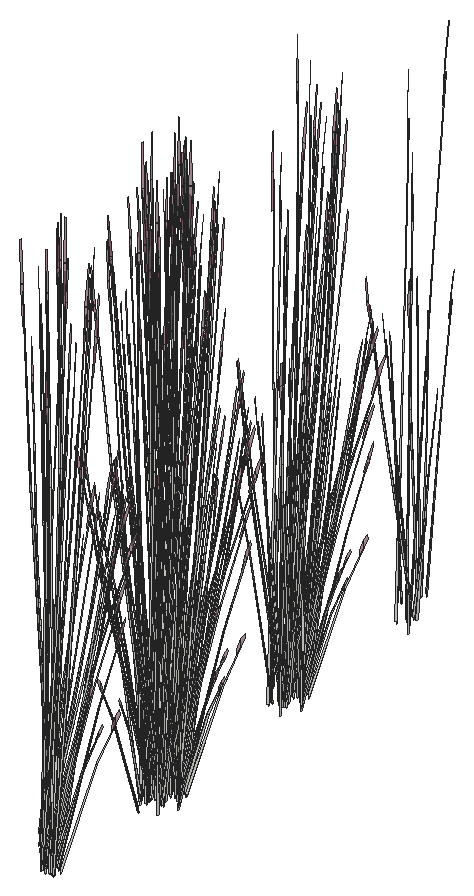
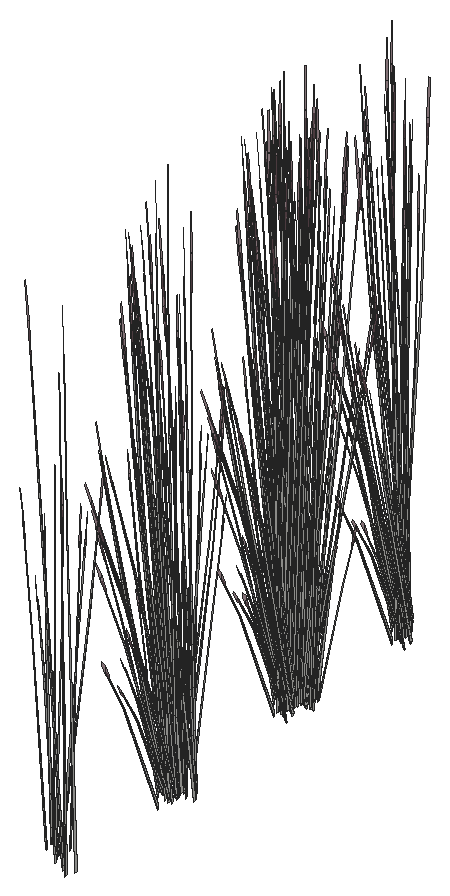
# SketchUp Ruby script. Lengths in inches.
U = 1.inch
M = Sketchup.active_model
def pt(a) = Geom::Point3d.new(a.map { |v| v * U })
def face(e, loops, mat)
  f = e.add_face(loops[0].map { |a| pt(a) })
  loops[1..].each { |l| e.add_face(l.map { |a| pt(a) }).erase! }
  f.material = f.back_material = mat if mat
  f
end
# faces: each face lists its corners as indices into pts; further lists are holes
def faces(e, pts, list, mat = nil) = list.each { |f| face(e, (f[0].is_a?(Array) ? f : [f]).map { |l| l.map { |i| pts[i] } }, mat) }
# xy, xz, yz: faces in a plane at the given z, y or x. An outline is a flat list of corners, or four numbers for a rectangle; further outlines are holes
def ring(l) = l.size == 4 ? [[l[0], l[1]], [l[2], l[1]], [l[2], l[3]], [l[0], l[3]]] : l.each_slice(2).to_a
def flat(e, list, mat, &to3) = list.each { |f| face(e, (f[0].is_a?(Array) ? f : [f]).map { |l| ring(l).map { |u, v| to3.(u, v) } }, mat) }
def xy(e, z, list, mat = nil) = flat(e, list, mat) { |x, y| [x, y, z] }
def xz(e, y, list, mat = nil) = flat(e, list, mat) { |x, z| [x, y, z] }
def yz(e, x, list, mat = nil) = flat(e, list, mat) { |y, z| [x, y, z] }
def lines(e, pts, list) = list.each { |a, b| e.add_line(pt(pts[a]), pt(pts[b])) }
# prism: a flat outline (further loops are holes) pulled along v
def prism(e, loops, v, mat = nil)
  f = face(e, loops, mat); d = Geom::Vector3d.new(v.map { |x| x * U })
  f.pushpull(f.normal.samedirection?(d) ? d.length : -d.length)
end
def box(e, o, s, mat = nil) = prism(e, [[o, [o[0] + s[0], o[1], o[2]], [o[0] + s[0], o[1] + s[1], o[2]], [o[0], o[1] + s[1], o[2]]]], [0, 0, s[2]], mat)
def at(x, y, z, deg = 0) = Geom::Transformation.translation(pt([x, y, z])) * Geom::Transformation.rotation(ORIGIN, Z_AXIS, deg.degrees)
def axes(o, x, y, z) = Geom::Transformation.new([*x, 0, *y, 0, *z, 0, *pt(o).to_a, 1])
def part(name) = M.definitions.add(name)
# library, detail: a bought-in or finely detailed component or shape, given as its bounding box
def library(name, o, s) = part(name).tap { |d| box(d.entities, o, s) }
def detail(e, o, s) = box(e.add_group.entities, o, s)
def put(e, d, t, mat = nil) = e.add_instance(d, t).tap { |i| i.material = mat if mat }
def group(e, t, mat = nil) = e.add_group.tap { |g| g.transformation = t; g.material = mat if mat }.entities
root = M.entities
M.materials.add("LightPink_Translucent").color = [144, 107, 117]
M.materials["LightPink_Translucent"].alpha = 0.75
c1 = part("blade")
p = [[2.15,0.21,22],[0,0.17,0],[0.09,0.45,0],[2.18,0.31,22],[2.29,0.31,22],[0.38,0.45,0],
  [2.48,0.24,33],[2.49,0.24,33],[2.48,0.22,33]]
faces(c1.entities,p,[[0,1,2,3],[4,5,2,3],[6,3,4,7],[8,0,3,6]])
c2 = part("seeds")
p = [[0.3,-0.1,1.38],[-0.01,-0.03,1.59],[-0.01,-0.03,0.03],[0.14,-0.07,-0.07],[0.29,-0.03,3],[0.15,0.01,3.11]]
faces(c2.entities,p,[[0,1,2,3],[1,0,4,5]],"LightPink_Translucent")
c3 = part("blade with seeds")
put(c3.entities,c1,at(0,0,0))
put(c3.entities,c2,axes([2.4,0.25,30.99],[1.5799,-0.05474,1.17369],[-0.12525,1.92788,0.29478],[-0.07173,-0.02425,1.56792]))
put(root,c3,axes([402.53,238.76,2.72],[0.38326,-0.02879,0.44739],[0.03466,0.47788,-0.21531],[-0.06861,0.04843,1.43643]))
put(root,c3,axes([402.77,238.28,2.62],[0.32884,-0.136,0.1448],[0.11516,0.38837,-0.41347],[0,0.08547,1.26744]))
put(root,c3,axes([403.99,239.22,2.59],[-0.085,-0.1147,1.43002],[0.1106,-0.37943,-0.30754],[0.17198,0.0514,0.61141]))
put(root,c3,axes([402.47,239.64,2.2],[0.35581,0.20937,0],[-0.17124,0.43505,0],[0,0,1.74954]))
put(root,c3,axes([402.61,240.1,2.19],[-0.21791,-0.46895,-0.05142],[0.36918,-0.26061,0.51607],[-0.09097,0.04465,1.6363]))
put(root,c3,axes([402.53,238.97,2.62],[0.26075,0.2802,0.1448],[-0.2175,0.31612,-0.41347],[-0.06054,0.04274,1.26744]))
put(root,c3,axes([403.21,239.45,4.98],[0.35281,0.01123,-0.71045],[-0.0237,0.47284,0.08574],[0.14947,0.0499,1.00501]))
put(root,c3,axes([402.8125,239.83,2.48],[0.33032,-0.23318,0.49651],[0.19744,0.41812,0],[-0.07523,0.05311,1.57504]))
put(root,c3,axes([402.34,239.46,2.29],[0.15345,0.53576,-0.06012],[-0.43845,0.18773,0],[0.00536,0.01871,1.72173]))
put(root,c3,axes([402.51,240.04,2.03],[-0.32928,-0.11539,-0.30978],[0.08291,-0.40636,0.30978],[-0.06638,0.04686,1.38974]))
put(root,c3,axes([403.78,238.49,2.375],[0.44133,0,0],[0,0.52122,-0.51607],[0,0.11871,1.63711]))
put(root,c3,axes([403.61,238.76,2.2],[-0.44111,-0.00373,-0.04976],[0,-0.52122,0.49943],[-0.01386,0.11865,1.58352]))
put(root,c3,axes([402.65,238.31,2.67],[0.39748,0.22252,-0.29095],[-0.19139,0.46966,-0.50002],[0.01249,0.11531,1.59708]))
put(root,c3,axes([403.42,239.65,4.53],[0.20082,0.29199,-0.35414],[-0.2293,0.2764,0.4572],[0.1165,0.04206,0.87481]))
put(root,c3,axes([403.52,238.84,2.03],[-0.24637,0.29097,-0.30978],[-0.24637,-0.29097,0.30978],[0,0.09372,1.38974]))
put(root,c3,axes([402.46,238.86,2.67],[0.04113,0.53214,-0.29095],[-0.42835,0.03218,-0.50002],[-0.07543,0.07088,1.59708]))
put(root,c3,axes([402.61,238.66,2.21],[-0.17124,0.42022,-0.44739],[-0.35581,-0.20224,0.21531],[0,0.09687,1.43643]))
put(root,c3,axes([402.62,239.86,2.33],[0.44186,0.15158,0.30756],[-0.11054,0.54181,-0.36492],[-0.07313,0.06781,1.64885]))
put(root,c3,axes([402.59,240.23,2.02],[-0.33032,0.23318,-0.49651],[-0.19744,-0.41812,0],[-0.07523,0.05311,1.57504]))
put(root,c3,axes([403.6875,238.85,2.02],[0,0.46636,-0.49651],[-0.39487,0,0],[0,0.10622,1.57504]))
put(root,c3,axes([402.7,238.9,3.875],[-0.1311,-0.08035,1.71376],[0.27131,-0.33708,0.13857],[0.16909,0.15206,0.73262]))
put(root,c3,axes([403.18,239.8125,2.77],[-0.19872,-0.13409,1.1486],[0.2566,-0.13625,0.84392],[0.06921,0.11541,0.25299]))
put(root,c3,axes([402.89,240.15,2.375],[0.22066,0.46731,0],[-0.36918,0.26061,-0.51607],[-0.08408,0.05936,1.63711]))
put(root,c3,axes([403.24,240.3125,1.49],[0.02571,-0.06733,1.76342],[0.32373,-0.19829,-0.26939],[0.09815,0.10263,0.30037]))
put(root,c3,axes([402.7,238.3,2.84],[-0.00964,-0.43909,1.41272],[0.43635,0.11382,0.59816],[-0.1032,0.24027,1.3335]))
put(root,c3,axes([402.8125,238.78,2.09],[0.12941,0.42699,-0.69212],[-0.37279,0.15378,-0.18165],[0.0143,0.14459,1.52773]))
put(root,c3,axes([402.74,240,4.68],[0.34827,-0.11086,-0.51099],[0.06092,0.41983,-0.3958],[0.09354,0.12031,0.97773]))
put(root,c3,axes([403.22,240.42,2.67],[-0.22633,-0.01463,1.0506],[0.14947,-0.31064,0.58006],[0.08941,0.11036,0.8241]))
put(root,c3,axes([402.48,239.67,2.59],[0.00623,-0.15459,1.43002],[0.29764,-0.17268,-0.30754],[0.09188,0.18503,0.61141]))
put(root,c3,axes([401.73,240.3,1.49],[0.05712,-0.02538,1.76342],[0.34359,0.13968,-0.26939],[0.01005,0.15742,0.30037]))
put(root,c3,axes([401.21,239.89,5],[0.25266,0.31335,-0.5672],[-0.2669,0.27442,-0.43934],[-0.03844,0.15921,1.08528]))
put(root,c3,axes([400.9375,240.36,2.82],[0.32063,-0.08258,0.06507],[0.07371,0.33271,-0.86304],[-0.02033,0.16842,0.7736]))
put(root,c3,axes([401.96,240.19,4.68],[0.34695,0.11691,-0.51099],[-0.11892,0.40083,-0.3958],[0.03181,0.16138,0.97773]))
put(root,c3,axes([402.16,239.37,3.875],[-0.08068,-0.14973,1.71376],[0.3728,-0.12606,0.13857],[0.08426,0.23506,0.73262]))
put(root,c3,axes([401.8,240.4375,4.53],[-0.1064,0.35863,-0.35414],[-0.31043,-0.1046,0.4572],[0.02846,0.14439,0.87481]))
put(root,c3,axes([401.5,239.44,3.875],[-0.00864,-0.17899,1.71376],[0.37441,0.11874,0.13857],[-0.02316,0.25508,0.73262]))
put(root,c3,axes([401.84,240.12,4.98],[0.16845,0.3792,-0.71045],[-0.34676,0.21133,0.08574],[0.03939,0.18322,1.00501]))
put(root,c3,axes([402.72,253.1,2.59],[-0.10032,0.0944,1.43002],[-0.30046,-0.16522,-0.30754],[0.05569,-0.20547,0.61141]))
put(root,c3,axes([402.27,253.42,4.98],[-0.16845,-0.3792,-0.71045],[0.34676,-0.21133,0.08574],[-0.03939,-0.18322,1.00501]))
put(root,c3,axes([401.98,252.58,1.49],[-0.0592,0.0168,1.76342],[-0.32738,-0.18913,-0.26939],[0.00549,-0.15776,0.30037]))
put(root,c3,axes([402.97,253.8,4.98],[0.00918,-0.43138,-0.71045],[0.38672,0.02897,0.08574],[0.04081,-0.18275,1.00501]))
put(root,c3,axes([402.3,253.1,4.53],[0.1064,-0.35863,-0.35414],[0.31043,0.1046,0.4572],[-0.02846,-0.14439,0.87481]))
put(root,c3,axes([402.53,253.58,3.875],[-0.06572,0.16029,1.71376],[-0.27569,-0.33172,0.13857],[0.12437,-0.20675,0.73262]))
put(root,c3,axes([402.14,253.35,4.68],[-0.34695,-0.11691,-0.51099],[0.11892,-0.40083,-0.3958],[-0.03181,-0.16138,0.97773]))
put(root,c3,axes([402.35,252.34,2.77],[0.04528,0.27194,1.1486],[-0.25117,-0.15062,0.84392],[0.02703,-0.13924,0.25299]))
put(root,c3,axes([402.89,253.65,4.68],[-0.25266,-0.31335,-0.51099],[0.2669,-0.27442,-0.3958],[0.03844,-0.15921,0.97773]))
put(root,c3,axes([403.13,253.54,4.53],[0.23881,-0.24554,-0.35414],[0.22606,0.28036,0.4572],[0.0344,-0.14245,0.87481]))
put(root,c3,axes([401.49,254.85,2.1],[-0.14494,-0.47823,-0.69835],[0.41752,-0.17223,-0.18329],[-0.01602,-0.16194,1.54149]))
put(root,c3,axes([403.43,253.39,1.49],[-0.05283,-0.03674,1.76342],[-0.13569,-0.41045,-0.26939],[0.09154,-0.11138,0.30037]))
put(root,c3,axes([403.42,254.55,4.98],[0.18436,-0.36797,-0.71045],[0.32306,0.26151,0.08574],[0.11008,-0.13332,1.00501]))
put(root,c3,axes([401.43,253.47,2.375],[-0.22066,-0.46731,0],[0.36918,-0.26061,-0.51607],[0.08408,-0.05936,1.63711]))
put(root,c3,axes([403.41,254.375,4.68],[-0.09067,-0.42583,-0.51099],[0.34336,-0.07449,-0.3958],[0.0984,-0.11438,0.97773]))
put(root,c3,axes([401.92,252.91,2.13],[-0.2439,0.26754,-0.03893],[-0.22348,-0.29302,-0.17649],[-0.01573,-0.08303,0.58215]))
put(root,c3,axes([400.63,254.78,2.02],[0,-0.46636,-0.49651],[0.39487,0,0],[0,-0.10622,1.57504]))
put(root,c3,axes([401.73,253.4,2.02],[0.33032,-0.23318,-0.49651],[0.19744,0.41812,0],[0.07523,-0.05311,1.57504]))
put(root,c3,axes([403.69,254.21,2.59],[-0.12609,-0.01381,1.43002],[-0.12917,-0.37055,-0.30754],[0.1549,-0.10482,0.61141]))
put(root,c3,axes([402.12,254.36,2.06],[0.23773,-0.35053,-0.62353],[0.29532,0.31785,-0.16365],[0.09526,-0.08744,1.37633]))
put(root,c3,axes([403.84,253.53,2.77],[-0.11756,0.2374,1.1486],[-0.10105,-0.31895,0.84392],[0.09709,-0.07992,0.25299]))
put(root,c3,axes([403.67,254.42,4.53],[0.30722,-0.06665,-0.35414],[0.08112,0.381,0.4572],[0.08804,-0.10234,0.87481]))
put(root,c3,axes([401.71,254.97,2.21],[0.17124,-0.42022,-0.44739],[0.35581,0.20224,0.21531],[0,-0.09687,1.43643]))
put(root,c3,axes([401.86,254.76,2.67],[-0.04113,-0.53214,-0.29095],[0.42835,-0.03218,-0.50002],[0.07543,-0.07088,1.59708]))
put(root,c3,axes([400.8,254.79,2.03],[0.24637,-0.29097,-0.30978],[0.24637,0.29097,0.30978],[0,-0.09372,1.38974]))
put(root,c3,axes([401.67,255.32,2.67],[-0.39748,-0.22252,-0.29095],[0.19139,-0.46966,-0.50002],[-0.01249,-0.11531,1.59708]))
put(root,c3,axes([401.81,253.59,2.03],[0.32928,0.11539,-0.30978],[-0.08291,0.40636,0.30978],[0.06638,-0.04686,1.38974]))
put(root,c3,axes([401.92,255.18,2.43],[0.39767,0.22603,0.24065],[-0.19139,0.46966,0.50002],[0,-0.10827,1.60543]))
put(root,c3,axes([401.77,255.82,2.4375],[0.09355,-0.55261,-0.23429],[0.44354,0.09633,0.51271],[-0.0775,-0.07631,1.5644]))
put(root,c3,axes([401.79,254.87,2.72],[-0.38326,0.02879,0.44739],[-0.03466,-0.47788,-0.21531],[0.06861,-0.04843,1.43643]))
put(root,c3,axes([400.8,255.22,2.48],[0,0.46636,0.49651],[-0.39487,0,0],[0,-0.10622,1.57504]))
put(root,c3,axes([403.57,255.32,4.68],[0.09562,-0.42421,-0.51099],[0.32782,0.1454,-0.3958],[0.13199,-0.0389,0.97773]))
put(root,c3,axes([403.06,253.59,2.375],[0.22066,-0.46731,0],[0.36918,0.26061,-0.51607],[0.08408,0.05936,1.63711]))
put(root,c3,axes([401.78,255.04,2.36],[0.15345,0.52148,0.45755],[-0.43845,0.18134,0.17955],[0.00536,-0.09582,1.58856]))
put(root,c3,axes([403.92,255.4375,1.98],[-0.22732,0.05597,1.41583],[-0.03618,-0.44548,0.08104],[0.15921,-0.06743,0.80566]))
put(root,c3,axes([404.34,255.04,2.26],[-0.21881,-0.29821,-0.06488],[0.23965,-0.27324,-0.29416],[0.0679,-0.01924,0.97024]))
put(root,c3,axes([401.7,255.45,2.72],[-0.17124,0.42022,0.44739],[-0.35581,-0.20224,-0.21531],[0,-0.09687,1.43643]))
put(root,c3,axes([402.33,255.08,2.21],[0,-0.53961,0],[0.44133,0,0],[0,0,1.79456]))
put(root,c3,axes([402.87,253.84,2.48],[-0.33032,-0.23318,0.49651],[0.19744,-0.41812,0],[0.07523,0.05311,1.57504]))
put(root,c3,axes([403.51,255.47,4.98],[0.31014,-0.20596,-0.71045],[0.17284,0.42397,0.08574],[0.14985,-0.04816,1.00501]))
put(root,c3,axes([402.12,254.74,2.36],[-0.29264,0.42323,0.45755],[-0.34767,-0.3736,0.17955],[0.07055,-0.04224,1.58856]))
put(root,c3,axes([402.44,255.5,2.3],[-0.32829,-0.4014,-0.06131],[0.32849,-0.40164,0],[-0.01146,-0.01402,1.75571]))
put(root,c3,axes([401.61,254.05,2.47],[-0.10196,0.46348,0.17642],[-0.3731,-0.13116,0.35086],[0.06445,-0.00226,1.60407]))
put(root,c3,axes([401.46,254.42,1.59],[-0.3474,0.18671,1.28929],[-0.11057,-0.53572,0.50096],[0.21332,0.00891,1.46642]))
put(root,c3,axes([402.39,254.5625,2.62],[0.06809,-0.4162,0.1448],[0.33266,0.07225,-0.41347],[0.06054,0.04274,1.26744]))
put(root,c3,axes([401.82,255.55,2.36],[0.44609,0.09826,0.45755],[-0.09078,0.55493,0.17955],[-0.06519,-0.05359,1.58856]))
put(root,c3,axes([404.17,255.15,1.49],[-0.01845,-0.0708,1.76342],[0.12793,-0.41416,-0.26939],[0.12905,-0.00596,0.30037]))
put(root,c3,axes([402.25,254.67,2.72],[-0.21202,-0.39143,0.44739],[0.32115,-0.27564,-0.21531],[0.06861,0.04843,1.43643]))
put(root,c3,axes([401.58,256.4375,2.47],[0.37926,-0.12378,0.17642],[0.09365,0.46065,0.35086],[-0.03382,-0.06712,1.60407]))
put(root,c3,axes([402.36,254.7,2.67],[0.35635,-0.30962,-0.29095],[0.23697,0.43749,-0.50002],[0.08792,0.04443,1.59708]))
put(root,c3,axes([403.78,255.51,4.53],[0.29332,0.1301,-0.35414],[-0.08555,0.37955,0.4572],[0.11809,-0.0348,0.87481]))
put(root,c3,axes([403.26,253.875,2.02],[0.33032,0.23318,-0.49651],[-0.19744,0.41812,0],[0.07523,0.05311,1.57504]))
put(root,c3,axes([402.63,255.2,2.21],[0.39487,0,0],[0,0.48281,0],[0,0,1.78407]))
put(root,c3,axes([402.74,254.07,2.47],[-0.37926,0.12378,0.17642],[-0.09365,-0.46065,0.35086],[0.03382,0.06712,1.60407]))
put(root,c3,axes([402.98,255.04,3.875],[-0.14639,0.01056,1.71376],[0.09712,-0.45778,0.13857],[0.20862,0.02831,0.73262]))
put(root,c3,axes([403.17,254.05,2.03],[0.08291,0.40636,-0.30978],[-0.32928,0.11539,0.30978],[0.06638,0.04686,1.38974]))
put(root,c3,axes([402.5,254.96,2.38],[-0.44609,-0.09826,0.49198],[0.09078,-0.55493,0.19306],[0.06519,0.05359,1.70813]))
put(root,c3,axes([402.15,256.33,2.2],[-0.11516,-0.40207,0],[0.32884,-0.1408,0],[0,0,1.54371]))
put(root,c3,axes([401.93,255.95,2.62],[-0.06809,0.4162,0.1448],[-0.33266,-0.07225,-0.41347],[-0.06054,-0.04274,1.26744]))
put(root,c3,axes([402.58,256.27,2.18],[0.37054,-0.15823,-0.19198],[0.1302,0.45581,0.00008],[0.0409,-0.01749,1.73897]))
put(root,c3,axes([402.71,256.46,2.47],[0.10196,-0.46348,0.17642],[0.3731,0.13116,0.35086],[-0.06445,0.00226,1.60407]))
put(root,c3,axes([402.62,255.41,2.21],[0.24637,0.30123,0],[-0.24637,0.30123,0],[0,0,1.69266]))
put(root,c3,axes([403.29,255.28,2.47],[-0.2773,-0.3397,0.17642],[0.27945,-0.32949,0.35086],[-0.03063,0.06937,1.60407]))
put(root,c3,axes([402.78,254.77,2.06],[0.36714,0.07646,-0.62353],[-0.07747,0.47163,-0.16365],[0.10956,0.05715,1.37633]))
put(root,c3,axes([404.4,255.59,2.77],[-0.21807,0.07699,1.1486],[0.10265,-0.31819,0.84392],[0.11568,0.02177,0.25299]))
put(root,c3,axes([402.07,256.51,2.2],[-0.35581,-0.20937,0],[0.17124,-0.43505,0],[0,0,1.62707]))
put(root,c3,axes([402.62,255.06,2.72],[0.17124,-0.42022,0.44739],[0.35581,0.20224,-0.21531],[0,0.09687,1.43643]))
put(root,c3,axes([402.55,255.3,2.29],[0,0.53934,-0.05637],[-0.44133,0,0],[0,0.01695,1.79368]))
put(root,c3,axes([402.58,254.92,2.21],[0.21202,0.39143,-0.44739],[-0.32115,0.27564,0.21531],[0.06861,0.04843,1.43643]))
put(root,c3,axes([404.02,256.57,3.93],[-0.06755,-0.39203,-0.03492],[0.31928,-0.09013,-0.15832],[0.06667,0.02485,0.52218]))
put(root,c3,axes([403.52,255.29,2.48],[0,-0.46636,0.49651],[0.39487,0,0],[0,0.10622,1.57504]))
put(root,c3,axes([402.53,255.64,2.72],[0.38326,-0.02879,0.44739],[0.03466,0.47788,-0.21531],[-0.06861,0.04843,1.43643]))
put(root,c3,axes([402.77,255.15,2.62],[0.32884,-0.136,0.1448],[0.11516,0.38837,-0.41347],[0,0.08547,1.26744]))
put(root,c3,axes([403.99,256.1,2.59],[-0.085,-0.1147,1.43002],[0.1106,-0.37943,-0.30754],[0.17198,0.0514,0.61141]))
put(root,c3,axes([402.47,256.52,2.2],[0.35581,0.20937,0],[-0.17124,0.43505,0],[0,0,1.74954]))
put(root,c3,axes([402.61,256.98,2.19],[-0.21791,-0.46895,-0.05142],[0.36918,-0.26061,0.51607],[-0.09097,0.04465,1.6363]))
put(root,c3,axes([402.53,255.85,2.62],[0.26075,0.2802,0.1448],[-0.2175,0.31612,-0.41347],[-0.06054,0.04274,1.26744]))
put(root,c3,axes([403.21,256.33,4.98],[0.35281,0.01123,-0.71045],[-0.0237,0.47284,0.08574],[0.14947,0.0499,1.00501]))
put(root,c3,axes([402.8125,256.71,2.48],[0.33032,-0.23318,0.49651],[0.19744,0.41812,0],[-0.07523,0.05311,1.57504]))
put(root,c3,axes([402.34,256.34,2.29],[0.15345,0.53576,-0.06012],[-0.43845,0.18773,0],[0.00536,0.01871,1.72173]))
put(root,c3,axes([402.51,256.92,2.03],[-0.32928,-0.11539,-0.30978],[0.08291,-0.40636,0.30978],[-0.06638,0.04686,1.38974]))
put(root,c3,axes([403.78,255.37,2.375],[0.44133,0,0],[0,0.52122,-0.51607],[0,0.11871,1.63711]))
put(root,c3,axes([403.61,255.64,2.2],[-0.44111,-0.00373,-0.04976],[0,-0.52122,0.49943],[-0.01386,0.11865,1.58352]))
put(root,c3,axes([402.65,255.19,2.67],[0.39748,0.22252,-0.29095],[-0.19139,0.46966,-0.50002],[0.01249,0.11531,1.59708]))
put(root,c3,axes([403.42,256.53,4.53],[0.20082,0.29199,-0.35414],[-0.2293,0.2764,0.4572],[0.1165,0.04206,0.87481]))
put(root,c3,axes([403.52,255.71,2.03],[-0.24637,0.29097,-0.30978],[-0.24637,-0.29097,0.30978],[0,0.09372,1.38974]))
put(root,c3,axes([402.46,255.74,2.67],[0.04113,0.53214,-0.29095],[-0.42835,0.03218,-0.50002],[-0.07543,0.07088,1.59708]))
put(root,c3,axes([402.61,255.53,2.21],[-0.17124,0.42022,-0.44739],[-0.35581,-0.20224,0.21531],[0,0.09687,1.43643]))
put(root,c3,axes([402.62,256.74,2.33],[0.44186,0.15158,0.30756],[-0.11054,0.54181,-0.36492],[-0.07313,0.06781,1.64885]))
put(root,c3,axes([402.59,257.11,2.02],[-0.33032,0.23318,-0.49651],[-0.19744,-0.41812,0],[-0.07523,0.05311,1.57504]))
put(root,c3,axes([403.6875,255.73,2.02],[0,0.46636,-0.49651],[-0.39487,0,0],[0,0.10622,1.57504]))
put(root,c3,axes([402.7,255.78,3.875],[-0.1311,-0.08035,1.71376],[0.27131,-0.33708,0.13857],[0.16909,0.15206,0.73262]))
put(root,c3,axes([403.18,256.69,2.77],[-0.19872,-0.13409,1.1486],[0.2566,-0.13625,0.84392],[0.06921,0.11541,0.25299]))
put(root,c3,axes([402.89,257.03,2.375],[0.22066,0.46731,0],[-0.36918,0.26061,-0.51607],[-0.08408,0.05936,1.63711]))
put(root,c3,axes([403.24,257.19,1.49],[0.02571,-0.06733,1.76342],[0.32373,-0.19829,-0.26939],[0.09815,0.10263,0.30037]))
put(root,c3,axes([402.7,255.18,2.84],[-0.00964,-0.43909,1.41272],[0.43635,0.11382,0.59816],[-0.1032,0.24027,1.3335]))
put(root,c3,axes([402.8125,255.66,2.09],[0.12941,0.42699,-0.69212],[-0.37279,0.15378,-0.18165],[0.0143,0.14459,1.52773]))
put(root,c3,axes([402.74,256.875,4.68],[0.34827,-0.11086,-0.51099],[0.06092,0.41983,-0.3958],[0.09354,0.12031,0.97773]))
put(root,c3,axes([403.22,257.3,2.67],[-0.22633,-0.01463,1.0506],[0.14947,-0.31064,0.58006],[0.08941,0.11036,0.8241]))
put(root,c3,axes([402.48,256.55,2.59],[0.00623,-0.15459,1.43002],[0.29764,-0.17268,-0.30754],[0.09188,0.18503,0.61141]))
put(root,c3,axes([401.73,257.18,1.49],[0.05712,-0.02538,1.76342],[0.34359,0.13968,-0.26939],[0.01005,0.15742,0.30037]))
put(root,c3,axes([401.21,256.77,5],[0.25266,0.31335,-0.5672],[-0.2669,0.27442,-0.43934],[-0.03844,0.15921,1.08528]))
put(root,c3,axes([400.9375,257.24,2.82],[0.32063,-0.08258,0.06507],[0.07371,0.33271,-0.86304],[-0.02033,0.16842,0.7736]))
put(root,c3,axes([401.96,257.07,4.68],[0.34695,0.11691,-0.51099],[-0.11892,0.40083,-0.3958],[0.03181,0.16138,0.97773]))
put(root,c3,axes([402.16,256.24,3.875],[-0.08068,-0.14973,1.71376],[0.3728,-0.12606,0.13857],[0.08426,0.23506,0.73262]))
put(root,c3,axes([401.8,257.32,4.53],[-0.1064,0.35863,-0.35414],[-0.31043,-0.1046,0.4572],[0.02846,0.14439,0.87481]))
put(root,c3,axes([401.5,256.32,3.875],[-0.00864,-0.17899,1.71376],[0.37441,0.11874,0.13857],[-0.02316,0.25508,0.73262]))
put(root,c3,axes([401.84,257,4.98],[0.16845,0.3792,-0.71045],[-0.34676,0.21133,0.08574],[0.03939,0.18322,1.00501]))
put(root,c3,axes([400.2,272.8,2.59],[-0.10032,0.0944,1.43002],[-0.30046,-0.16522,-0.30754],[0.05569,-0.20547,0.61141]))
put(root,c3,axes([400.45,273.5,4.98],[0.00918,-0.43138,-0.71045],[0.38672,0.02897,0.08574],[0.04081,-0.18275,1.00501]))
put(root,c3,axes([400.01,273.28,3.875],[-0.06572,0.16029,1.71376],[-0.27569,-0.33172,0.13857],[0.12437,-0.20675,0.73262]))
put(root,c3,axes([400.37,273.35,4.68],[-0.25266,-0.31335,-0.51099],[0.2669,-0.27442,-0.3958],[0.03844,-0.15921,0.97773]))
put(root,c3,axes([400.61,273.24,4.53],[0.23881,-0.24554,-0.35414],[0.22606,0.28036,0.4572],[0.0344,-0.14245,0.87481]))
put(root,c3,axes([400.9,273.09,1.49],[-0.05283,-0.03674,1.76342],[-0.13569,-0.41045,-0.26939],[0.09154,-0.11138,0.30037]))
put(root,c3,axes([400.9,274.25,4.98],[0.18436,-0.36797,-0.71045],[0.32306,0.26151,0.08574],[0.11008,-0.13332,1.00501]))
put(root,c3,axes([400.89,274.08,4.68],[-0.09067,-0.42583,-0.51099],[0.34336,-0.07449,-0.3958],[0.0984,-0.11438,0.97773]))
put(root,c3,axes([399.21,273.1,2.02],[0.33032,-0.23318,-0.49651],[0.19744,0.41812,0],[0.07523,-0.05311,1.57504]))
put(root,c3,axes([401.17,273.91,2.59],[-0.12609,-0.01381,1.43002],[-0.12917,-0.37055,-0.30754],[0.1549,-0.10482,0.61141]))
put(root,c3,axes([399.6,274.06,2.06],[0.23773,-0.35053,-0.62353],[0.29532,0.31785,-0.16365],[0.09526,-0.08744,1.37633]))
put(root,c3,axes([401.3125,273.23,2.77],[-0.11756,0.2374,1.1486],[-0.10105,-0.31895,0.84392],[0.09709,-0.07992,0.25299]))
put(root,c3,axes([401.15,274.12,4.53],[0.30722,-0.06665,-0.35414],[0.08112,0.381,0.4572],[0.08804,-0.10234,0.87481]))
put(root,c3,axes([399.34,274.47,2.67],[-0.04113,-0.53214,-0.29095],[0.42835,-0.03218,-0.50002],[0.07543,-0.07088,1.59708]))
put(root,c3,axes([399.29,273.29,2.03],[0.32928,0.11539,-0.30978],[-0.08291,0.40636,0.30978],[0.06638,-0.04686,1.38974]))
put(root,c3,axes([401.05,275.02,4.68],[0.09562,-0.42421,-0.51099],[0.32782,0.1454,-0.3958],[0.13199,-0.0389,0.97773]))
put(root,c3,axes([400.53,273.29,2.375],[0.22066,-0.46731,0],[0.36918,0.26061,-0.51607],[0.08408,0.05936,1.63711]))
put(root,c3,axes([401.4,275.14,1.98],[-0.22732,0.05597,1.41583],[-0.03618,-0.44548,0.08104],[0.15921,-0.06743,0.80566]))
put(root,c3,axes([401.82,274.75,2.26],[-0.21881,-0.29821,-0.06488],[0.23965,-0.27324,-0.29416],[0.0679,-0.01924,0.97024]))
put(root,c3,axes([400.34,273.54,2.48],[-0.33032,-0.23318,0.49651],[0.19744,-0.41812,0],[0.07523,0.05311,1.57504]))
put(root,c3,axes([400.99,275.18,4.98],[0.31014,-0.20596,-0.71045],[0.17284,0.42397,0.08574],[0.14985,-0.04816,1.00501]))
put(root,c3,axes([398.9375,274.12,1.59],[-0.3474,0.18671,1.28929],[-0.11057,-0.53572,0.50096],[0.21332,0.00891,1.46642]))
put(root,c3,axes([399.87,274.26,2.62],[0.06809,-0.4162,0.1448],[0.33266,0.07225,-0.41347],[0.06054,0.04274,1.26744]))
put(root,c3,axes([401.65,274.85,1.49],[-0.01845,-0.0708,1.76342],[0.12793,-0.41416,-0.26939],[0.12905,-0.00596,0.30037]))
put(root,c3,axes([399.73,274.37,2.72],[-0.21202,-0.39143,0.44739],[0.32115,-0.27564,-0.21531],[0.06861,0.04843,1.43643]))
put(root,c3,axes([399.84,274.4,2.67],[0.35635,-0.30962,-0.29095],[0.23697,0.43749,-0.50002],[0.08792,0.04443,1.59708]))
put(root,c3,axes([401.25,275.21,4.53],[0.29332,0.1301,-0.35414],[-0.08555,0.37955,0.4572],[0.11809,-0.0348,0.87481]))
put(root,c3,axes([400.73,273.57,2.02],[0.33032,0.23318,-0.49651],[-0.19744,0.41812,0],[0.07523,0.05311,1.57504]))
put(root,c3,axes([400.11,274.91,2.21],[0.39487,0,0],[0,0.48281,0],[0,0,1.78407]))
put(root,c3,axes([400.45,274.74,3.875],[-0.14639,0.01056,1.71376],[0.09712,-0.45778,0.13857],[0.20862,0.02831,0.73262]))
put(root,c3,axes([400.64,273.75,2.03],[0.08291,0.40636,-0.30978],[-0.32928,0.11539,0.30978],[0.06638,0.04686,1.38974]))
put(root,c3,axes([400.06,275.97,2.18],[0.37054,-0.15823,-0.19198],[0.1302,0.45581,0.00008],[0.0409,-0.01749,1.73897]))
put(root,c3,axes([400.25,274.47,2.06],[0.36714,0.07646,-0.62353],[-0.07747,0.47163,-0.16365],[0.10956,0.05715,1.37633]))
put(root,c3,axes([401.875,275.29,2.77],[-0.21807,0.07699,1.1486],[0.10265,-0.31819,0.84392],[0.11568,0.02177,0.25299]))
put(root,c3,axes([400.0625,274.62,2.21],[0.21202,0.39143,-0.44739],[-0.32115,0.27564,0.21531],[0.06861,0.04843,1.43643]))
put(root,c3,axes([401.5,276.27,3.93],[-0.06755,-0.39203,-0.03492],[0.31928,-0.09013,-0.15832],[0.06667,0.02485,0.52218]))
put(root,c3,axes([400.99,274.99,2.48],[0,-0.46636,0.49651],[0.39487,0,0],[0,0.10622,1.57504]))
put(root,c3,axes([400.24,274.86,2.62],[0.32884,-0.136,0.1448],[0.11516,0.38837,-0.41347],[0,0.08547,1.26744]))
put(root,c3,axes([401.47,275.8,2.59],[-0.085,-0.1147,1.43002],[0.1106,-0.37943,-0.30754],[0.17198,0.0514,0.61141]))
put(root,c3,axes([400.6875,276.03,4.98],[0.35281,0.01123,-0.71045],[-0.0237,0.47284,0.08574],[0.14947,0.0499,1.00501]))
put(root,c3,axes([401.26,275.07,2.375],[0.44133,0,0],[0,0.52122,-0.51607],[0,0.11871,1.63711]))
put(root,c3,axes([400.13,274.89,2.67],[0.39748,0.22252,-0.29095],[-0.19139,0.46966,-0.50002],[0.01249,0.11531,1.59708]))
put(root,c3,axes([400.9,276.23,4.53],[0.20082,0.29199,-0.35414],[-0.2293,0.2764,0.4572],[0.1165,0.04206,0.87481]))
put(root,c3,axes([401.16,275.43,2.02],[0,0.46636,-0.49651],[-0.39487,0,0],[0,0.10622,1.57504]))
put(root,c3,axes([400.18,275.48,3.875],[-0.1311,-0.08035,1.71376],[0.27131,-0.33708,0.13857],[0.16909,0.15206,0.73262]))
put(root,c3,axes([400.66,276.39,2.77],[-0.19872,-0.13409,1.1486],[0.2566,-0.13625,0.84392],[0.06921,0.11541,0.25299]))
put(root,c3,axes([400.72,276.89,1.49],[0.02571,-0.06733,1.76342],[0.32373,-0.19829,-0.26939],[0.09815,0.10263,0.30037]))
put(root,c3,axes([400.29,275.36,2.09],[0.12941,0.42699,-0.69212],[-0.37279,0.15378,-0.18165],[0.0143,0.14459,1.52773]))
put(root,c3,axes([400.21,276.58,4.68],[0.34827,-0.11086,-0.51099],[0.06092,0.41983,-0.3958],[0.09354,0.12031,0.97773]))
put(root,c3,axes([400.69,277,2.67],[-0.22633,-0.01463,1.0506],[0.14947,-0.31064,0.58006],[0.08941,0.11036,0.8241]))
put(root,c3,axes([399.96,276.25,2.59],[0.00623,-0.15459,1.43002],[0.29764,-0.17268,-0.30754],[0.09188,0.18503,0.61141]))
put(root,c3,axes([399.64,275.95,3.875],[-0.08068,-0.14973,1.71376],[0.3728,-0.12606,0.13857],[0.08426,0.23506,0.73262]))
put(root,c3,axes([400,291.26,4.98],[0.00918,-0.43138,-0.71045],[0.38672,0.02897,0.08574],[0.04081,-0.18275,1.00501]))
put(root,c3,axes([399.56,291.04,3.875],[-0.06572,0.16029,1.71376],[-0.27569,-0.33172,0.13857],[0.12437,-0.20675,0.73262]))
put(root,c3,axes([400.16,291,4.53],[0.23881,-0.24554,-0.35414],[0.22606,0.28036,0.4572],[0.0344,-0.14245,0.87481]))
put(root,c3,axes([400.46,290.85,1.49],[-0.05283,-0.03674,1.76342],[-0.13569,-0.41045,-0.26939],[0.09154,-0.11138,0.30037]))
put(root,c3,axes([400.46,292.01,4.98],[0.18436,-0.36797,-0.71045],[0.32306,0.26151,0.08574],[0.11008,-0.13332,1.00501]))
put(root,c3,axes([400.45,291.84,4.68],[-0.09067,-0.42583,-0.51099],[0.34336,-0.07449,-0.3958],[0.0984,-0.11438,0.97773]))
put(root,c3,axes([398.76,290.87,2.02],[0.33032,-0.23318,-0.49651],[0.19744,0.41812,0],[0.07523,-0.05311,1.57504]))
put(root,c3,axes([400.72,291.67,2.59],[-0.12609,-0.01381,1.43002],[-0.12917,-0.37055,-0.30754],[0.1549,-0.10482,0.61141]))
put(root,c3,axes([399.15,291.82,2.06],[0.23773,-0.35053,-0.62353],[0.29532,0.31785,-0.16365],[0.09526,-0.08744,1.37633]))
put(root,c3,axes([400.87,290.99,2.77],[-0.11756,0.2374,1.1486],[-0.10105,-0.31895,0.84392],[0.09709,-0.07992,0.25299]))
put(root,c3,axes([400.7,291.88,4.53],[0.30722,-0.06665,-0.35414],[0.08112,0.381,0.4572],[0.08804,-0.10234,0.87481]))
put(root,c3,axes([400.61,292.78,4.68],[0.09562,-0.42421,-0.51099],[0.32782,0.1454,-0.3958],[0.13199,-0.0389,0.97773]))
put(root,c3,axes([400.09,291.06,2.375],[0.22066,-0.46731,0],[0.36918,0.26061,-0.51607],[0.08408,0.05936,1.63711]))
